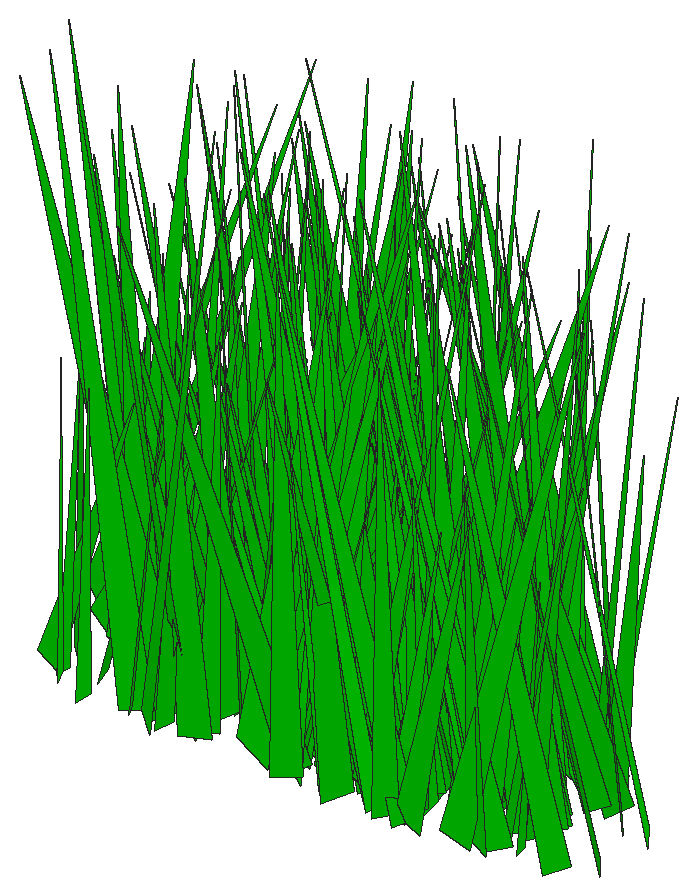
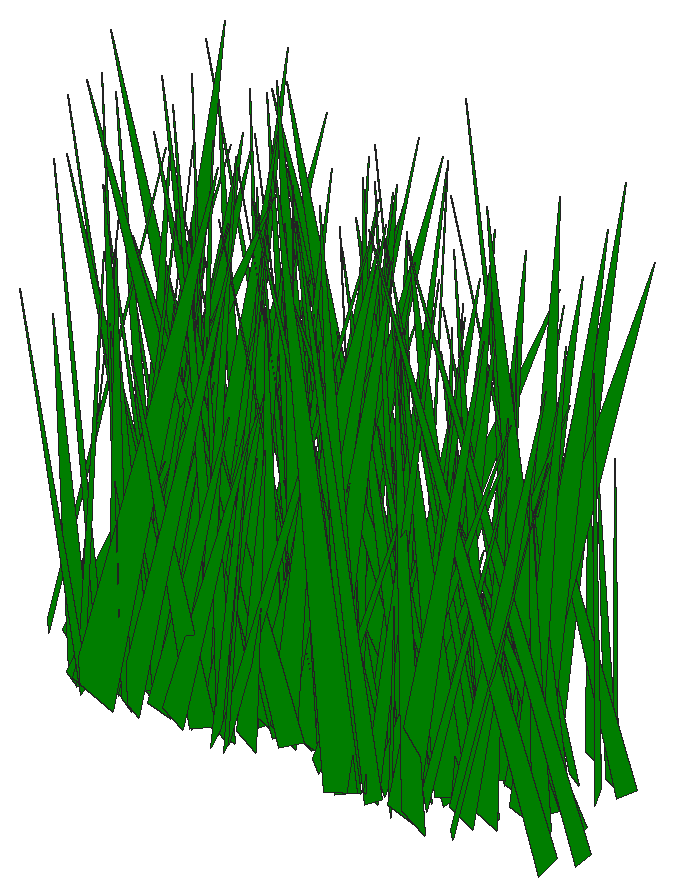
# SketchUp Ruby script. Lengths in inches.
U = 1.inch
M = Sketchup.active_model
def pt(a) = Geom::Point3d.new(a.map { |v| v * U })
def face(e, loops, mat)
  f = e.add_face(loops[0].map { |a| pt(a) })
  loops[1..].each { |l| e.add_face(l.map { |a| pt(a) }).erase! }
  f.material = f.back_material = mat if mat
  f
end
# faces: each face lists its corners as indices into pts; further lists are holes
def faces(e, pts, list, mat = nil) = list.each { |f| face(e, (f[0].is_a?(Array) ? f : [f]).map { |l| l.map { |i| pts[i] } }, mat) }
# xy, xz, yz: faces in a plane at the given z, y or x. An outline is a flat list of corners, or four numbers for a rectangle; further outlines are holes
def ring(l) = l.size == 4 ? [[l[0], l[1]], [l[2], l[1]], [l[2], l[3]], [l[0], l[3]]] : l.each_slice(2).to_a
def flat(e, list, mat, &to3) = list.each { |f| face(e, (f[0].is_a?(Array) ? f : [f]).map { |l| ring(l).map { |u, v| to3.(u, v) } }, mat) }
def xy(e, z, list, mat = nil) = flat(e, list, mat) { |x, y| [x, y, z] }
def xz(e, y, list, mat = nil) = flat(e, list, mat) { |x, z| [x, y, z] }
def yz(e, x, list, mat = nil) = flat(e, list, mat) { |y, z| [x, y, z] }
def lines(e, pts, list) = list.each { |a, b| e.add_line(pt(pts[a]), pt(pts[b])) }
# prism: a flat outline (further loops are holes) pulled along v
def prism(e, loops, v, mat = nil)
  f = face(e, loops, mat); d = Geom::Vector3d.new(v.map { |x| x * U })
  f.pushpull(f.normal.samedirection?(d) ? d.length : -d.length)
end
def box(e, o, s, mat = nil) = prism(e, [[o, [o[0] + s[0], o[1], o[2]], [o[0] + s[0], o[1] + s[1], o[2]], [o[0], o[1] + s[1], o[2]]]], [0, 0, s[2]], mat)
def at(x, y, z, deg = 0) = Geom::Transformation.translation(pt([x, y, z])) * Geom::Transformation.rotation(ORIGIN, Z_AXIS, deg.degrees)
def axes(o, x, y, z) = Geom::Transformation.new([*x, 0, *y, 0, *z, 0, *pt(o).to_a, 1])
def part(name) = M.definitions.add(name)
# library, detail: a bought-in or finely detailed component or shape, given as its bounding box
def library(name, o, s) = part(name).tap { |d| box(d.entities, o, s) }
def detail(e, o, s) = box(e.add_group.entities, o, s)
def put(e, d, t, mat = nil) = e.add_instance(d, t).tap { |i| i.material = mat if mat }
def group(e, t, mat = nil) = e.add_group.tap { |g| g.transformation = t; g.material = mat if mat }.entities
root = M.entities
M.materials.add("[Color G06]").color = [0, 204, 0]
c1 = part("fur_instance\#9")
p = [[0.8125,0,1.79],[0.67,-0.02,1.48],[0,-0.11,0],[0,0.11,0]]
faces(c1.entities,p,[[0,1,2,3]])
put(root,c1,axes([93.32,20.96,4.28],[-4.15856,-0.04522,0.42763],[-0.24087,0.56256,1.60087],[0.35916,-0.14626,6.02509]),"[Color G06]")
put(root,c1,axes([93.11,18.42,4.28],[-1.77363,-0.76487,1.40268],[-5.54361,0.23087,-1.19607],[-0.48553,0.1581,8.53241]),"[Color G06]")
put(root,c1,axes([92.51,19.21,4.28],[-3.03787,0.38662,3.31742],[3.46807,0.41073,1.5953],[0.76567,-0.32643,5.93635]),"[Color G06]")
put(root,c1,axes([91.73,17.29,4.28],[-3.61596,-0.26712,1.95596],[-1.26486,0.5103,2.78243],[1.94484,-0.16477,5.44624]),"[Color G06]")
put(root,c1,axes([91.68,19.55,4.28],[-1.50021,-0.43243,0.52191],[-2.93541,0.21388,1.50933],[1.05913,-0.01973,4.9224]),"[Color G06]")
put(root,c1,axes([91.92,16.38,4.28],[-2.78396,-0.01619,2.16058],[0.38948,0.41195,1.47567],[1.397,-0.14712,3.89424]),"[Color G06]")
put(root,c1,axes([91.82,16.63,4.28],[2.58132,-0.22761,0.58761],[-1.48872,-0.35679,-1.26735],[-0.77617,-0.07262,4.38507]),"[Color G06]")
put(root,c1,axes([92.02,18.39,4.28],[-1.45035,0.39442,0.16935],[2.67143,0.19658,-1.48927],[0.93634,0.05009,4.5113]),"[Color G06]")
put(root,c1,axes([93.66,20.17,4.28],[-2.8666,-0.46823,1.58178],[-3.517,0.37218,-1.58151],[-0.16044,0.20749,6.40624]),"[Color G06]")
put(root,c1,axes([93.95,17.52,4.28],[0.25229,0.76715,0.79622],[5.25095,-0.05648,2.53488],[-1.7254,-0.05972,7.83087]),"[Color G06]")
put(root,c1,axes([91.25,16.77,4.28],[0.7768,-0.41726,0.47828],[-2.7764,-0.08159,1.89573],[1.16095,0.08407,4.21362]),"[Color G06]")
put(root,c1,axes([95.05,16.57,4.28],[-1.07004,0.80814,0.91519],[5.3939,0.10448,3.48938],[-2.20617,-0.13653,8.08736]),"[Color G06]")
put(root,c1,axes([93.05,17.76,4.28],[-2.5649,0.23425,0.39401],[1.54825,0.34923,-1.33748],[0.70304,0.08551,4.38288]),"[Color G06]")
put(root,c1,axes([90.93,19.04,4.28],[2.31582,-0.30652,0.01263],[-1.93543,-0.28352,2.27407],[1.04211,0.1546,4.19539]),"[Color G06]")
put(root,c1,axes([90.05,19.96,4.28],[5.14354,0.39233,0.20234],[2.70873,-0.67815,-2.75667],[0.77264,-0.23431,8.31738]),"[Color G06]")
put(root,c1,axes([94.3,16.24,4.28],[-3.81085,0.59634,1.81684],[4.44015,0.52185,1.127],[0.2262,-0.19697,8.48654]),"[Color G06]")
put(root,c1,axes([93.15,19.87,4.28],[2.44916,-0.44573,0.93395],[-2.98196,-0.35073,-1.7608],[-1.3098,-0.03497,5.75509]),"[Color G06]")
put(root,c1,axes([90.51,20.76,4.28],[5.74425,-0.28536,0.29791],[-2.01718,-0.7662,2.57285],[0.39787,0.2352,8.743]),"[Color G06]")
put(root,c1,axes([92.99,15.9,4.28],[2.57562,-0.26491,0.59469],[-1.71125,-0.35343,-1.53066],[-0.91598,-0.08461,4.53179]),"[Color G06]")
put(root,c1,axes([92.71,18.14,4.28],[-2.36462,0.75183,1.28791],[5.14929,0.35062,-2.39404],[1.81562,-0.01522,8.46708]),"[Color G06]")
put(root,c1,axes([94.37,17.5,4.28],[1.53115,-0.71337,0.51031],[-4.83016,-0.21736,-2.53265],[-1.71957,-0.02464,7.56846]),"[Color G06]")
put(root,c1,axes([94.9,20.03,4.28],[-3.81415,-0.1096,0.77234],[-0.93183,0.48136,-2.43211],[0.1285,0.23741,5.28779]),"[Color G06]")
put(root,c1,axes([94.87,20.97,4.28],[-3.38658,0.46529,1.95903],[3.5822,0.44899,1.58233],[0.13948,-0.23415,6.92708]),"[Color G06]")
put(root,c1,axes([94.38,16.61,4.28],[1.06724,0.74929,1.90632],[5.40058,-0.17948,1.3503],[-1.15494,-0.14687,8.07567]),"[Color G06]")
put(root,c1,axes([93.25,19.56,4.28],[4.75611,-0.26276,1.8293],[-1.75691,-0.68397,-1.08237],[-1.40073,-0.0343,7.56892]),"[Color G06]")
put(root,c1,axes([96.21,20.11,4.28],[-4.19539,-0.22607,0.18995],[-1.56836,0.54953,-2.24485],[-0.42988,0.20147,6.33629]),"[Color G06]")
put(root,c1,axes([96.22,17.75,4.28],[-3.63597,-0.30668,0.22846],[-2.1222,0.47577,-2.07945],[-0.59697,0.17654,6.00089]),"[Color G06]")
put(root,c1,axes([94.35,17.47,4.28],[3.6807,0.05354,2.82113],[0.94083,-0.54532,-1.55298],[-1.68084,-0.18799,5.30843]),"[Color G06]")
put(root,c1,axes([95.64,17.23,4.28],[-1.1041,0.3479,1.4162],[2.57625,0.10162,1.61887],[-0.6966,-0.17561,3.74247]),"[Color G06]")
put(root,c1,axes([94.19,16.15,4.28],[3.40681,0.14764,1.18837],[0.80818,-0.4743,1.59383],[-1.04883,0.11409,5.08817]),"[Color G06]")
put(root,c1,axes([92.7,16.99,4.28],[5.49237,-0.09231,0.12074],[-0.63393,-0.75171,-1.6022],[-0.20697,-0.14711,8.11144]),"[Color G06]")
put(root,c1,axes([96.08,18.93,4.28],[-0.04304,0.39725,0.22765],[2.53975,-0.00434,1.94263],[-1.29945,-0.02164,3.78929]),"[Color G06]")
put(root,c1,axes([93.62,17.48,4.28],[4.23265,-0.12896,1.03424],[-1.06102,-0.57897,1.40614],[-0.45653,0.1499,6.32074]),"[Color G06]")
put(root,c1,axes([95.92,16.22,4.28],[-3.92501,-0.29525,0.5518],[-2.03835,0.54535,1.13373],[0.68158,-0.06933,6.56821]),"[Color G06]")
put(root,c1,axes([94.42,21.09,4.28],[3.80061,-0.41677,0.32666],[-2.77508,-0.50805,-2.33923],[-1.13103,-0.15391,6.83716]),"[Color G06]")
put(root,c1,axes([95.98,20.77,4.28],[-4.91749,0.15917,2.11364],[1.41638,0.6921,1.37353],[1.13877,-0.17348,7.41888]),"[Color G06]")
put(root,c1,axes([96.0625,19.18,4.28],[-4.84141,0.19014,0.95387],[1.11253,0.65377,-2.35708],[1.01431,0.19047,7.13825]),"[Color G06]")
put(root,c1,axes([95.21,19.43,4.28],[2.71413,-0.27368,1.71108],[-1.75241,-0.41044,-1.33229],[-1.44627,-0.01628,4.82537]),"[Color G06]")
put(root,c1,axes([94.52,19.5,4.28],[-0.67718,0.63406,0.19879],[4.44886,0.09622,-1.40461],[0.94912,0.00136,6.72572]),"[Color G06]")
put(root,c1,axes([93.79,19.0625,4.28],[5.0228,0.35797,0.25556],[2.43856,-0.67907,2.20981],[-0.82013,0.1732,8.1358]),"[Color G06]")
put(root,c1,axes([96,18.0625,4.28],[-0.22793,0.54055,2.68699],[4.18813,-0.02154,1.29143],[-0.84767,-0.25179,5.65813]),"[Color G06]")
put(root,c1,axes([94.15,18.125,4.28],[0.89299,-0.56458,0.06541],[-3.97459,-0.12104,1.19653],[0.77259,0.02989,6.07996]),"[Color G06]")
put(root,c1,axes([96.78,18.86,4.28],[2.44031,0.64518,2.4293],[4.02432,-0.40814,3.42196],[-2.80248,-0.02428,7.02925]),"[Color G06]")
put(root,c1,axes([95.33,20.85,4.28],[4.3793,-0.07884,2.83715],[0.27014,-0.61257,-2.88679],[-1.96219,-0.26028,5.93464]),"[Color G06]")
put(root,c1,axes([94.95,19.85,4.28],[3.02987,0.20285,0.89994],[1.31134,-0.42593,1.16666],[-0.87121,0.06434,4.88586]),"[Color G06]")
put(root,c1,axes([95.29,16.05,4.28],[3.25163,0.45455,0.54285],[3.00175,-0.44117,2.27195],[-1.3217,0.11632,6.49542]),"[Color G06]")
put(root,c1,axes([96.18,16.07,4.28],[0.17155,0.64687,1.77041],[4.70831,-0.05278,1.19617],[-0.86854,-0.15834,6.83401]),"[Color G06]")
put(root,c1,axes([94.76,18.55,4.28],[-1.60592,0.64467,2.18363],[4.5724,0.27276,-1.73896],[1.61269,-0.13138,7.10484]),"[Color G06]")
put(root,c1,axes([96.01,17.88,4.28],[-2.75426,0.29226,0.22472],[1.9301,0.36555,-1.77091],[0.83062,0.11968,4.86014]),"[Color G06]")
put(root,c1,axes([97.33,18.375,4.28],[-1.28275,-0.46751,0.11305],[-3.08854,0.1603,-2.13],[-1.30655,0.08007,4.92411]),"[Color G06]")
put(root,c1,axes([94.08,17.98,4.28],[4.007,0.04567,0.15646],[0.34235,-0.51403,-2.34831],[0.032,-0.21954,5.53085]),"[Color G06]")
put(root,c1,axes([96.22,17.62,4.28],[2.95874,-0.67113,0.30492],[-4.43795,-0.39275,-3.11048],[-1.87344,-0.12955,7.8499]),"[Color G06]")
put(root,c1,axes([95.78,18.22,4.28],[2.745,-0.41858,1.48213],[-2.89887,-0.40634,-1.1901],[-1.26111,0.02295,5.96172]),"[Color G06]")
put(root,c1,axes([94.83,15.92,4.28],[5.53723,0.18183,2.45849],[1.71203,-0.76564,-2.1082],[-1.21456,-0.25024,8.23666]),"[Color G06]")
put(root,c1,axes([95.15,19.18,4.28],[0.54778,-0.44335,1.12213],[-3.15104,-0.04369,1.45299],[0.86211,0.12201,4.59774]),"[Color G06]")
put(root,c1,axes([96.51,18.26,4.28],[-5.34507,-0.08397,2.94885],[-0.23534,0.78396,1.61168],[2.04942,-0.12898,7.87593]),"[Color G06]")
put(root,c1,axes([96.71,17.15,4.28],[-4.08381,-0.02123,2.1514],[-0.52777,0.58131,-1.57891],[1.34786,0.1633,5.90019]),"[Color G06]")
put(root,c1,axes([96.29,16.45,4.28],[1.64611,0.4765,0.34657],[3.34245,-0.23133,1.07397],[-0.7474,0.01496,5.56619]),"[Color G06]")
put(root,c1,axes([97.29,18.92,4.28],[-5.45701,0.17626,3.29785],[2.063,0.73278,3.1261],[1.48684,-0.36981,7.7663]),"[Color G06]")
put(root,c1,axes([99.04,16.33,4.28],[-2.73396,-0.61043,0.12845],[-4.05016,0.34722,-3.00448],[-1.66336,0.15787,7.10459]),"[Color G06]")
put(root,c1,axes([98.01,20.36,4.28],[-3.30955,-0.16179,0.09083],[-1.13461,0.44458,-1.37871],[-0.2499,0.12412,5.05692]),"[Color G06]")
put(root,c1,axes([97.95,17.62,4.28],[-2.79481,0.18158,0.23896],[1.2752,0.36367,1.5706],[-0.30815,-0.14186,4.33224]),"[Color G06]")
put(root,c1,axes([97.9,17.74,4.28],[-1.4915,-0.42185,1.28772],[-3.04073,0.15934,-1.87086],[-0.805,0.17973,4.68099]),"[Color G06]")
put(root,c1,axes([95.625,19.05,4.28],[0.95502,0.50004,1.12401],[3.58865,-0.10581,-1.40371],[0.73877,-0.13243,5.36562]),"[Color G06]")
put(root,c1,axes([95.4,19.8,4.28],[4.65554,-0.32798,0.29399],[-2.27103,-0.639,-1.55929],[-0.64281,-0.11783,7.63809]),"[Color G06]")
put(root,c1,axes([94.38,19.51,4.28],[3.04406,0.5202,0.87894],[3.48315,-0.34602,-3.421],[1.45953,-0.25919,6.33101]),"[Color G06]")
put(root,c1,axes([98.27,17.75,4.28],[-1.95236,-0.34271,0.83146],[-2.47148,0.24129,-1.53797],[-0.49138,0.14803,4.43185]),"[Color G06]")
put(root,c1,axes([96.49,18.89,4.28],[5.06297,-0.18053,2.25382],[-1.06562,-0.73234,-1.39143],[-1.67767,-0.07965,7.68551]),"[Color G06]")
put(root,c1,axes([95.81,20.88,4.28],[4.49793,0.34569,2.2561],[2.83354,-0.6071,-1.93267],[-0.62885,-0.26293,7.42864]),"[Color G06]")
put(root,c1,axes([96.76,20.5,4.28],[-3.58448,0.56107,2.40881],[3.82919,0.54656,-1.89621],[2.03075,-0.04026,7.82732]),"[Color G06]")
put(root,c1,axes([96.59,20.99,4.28],[-0.73322,-0.45925,0.49484],[-3.15637,0.11125,1.4137],[0.99678,0.01446,4.84056]),"[Color G06]")
put(root,c1,axes([98.7,19.42,4.28],[0.70035,0.68534,2.16868],[4.82518,-0.15697,2.21758],[-1.72572,-0.16075,7.08055]),"[Color G06]")
put(root,c1,axes([97.58,19.45,4.28],[2.44316,-0.35319,1.3697],[-2.39262,-0.36382,-1.24386],[-1.23718,0.00611,5.11042]),"[Color G06]")
put(root,c1,axes([97.16,19.55,4.28],[4.77282,0.02242,2.53589],[0.59937,-0.68069,-1.82859],[-1.59546,-0.18865,6.89916]),"[Color G06]")
put(root,c1,axes([98.23,17.1,4.28],[1.16702,0.45356,0.2273],[3.04665,-0.16005,1.74612],[-1.14906,0.03629,4.86054]),"[Color G06]")
put(root,c1,axes([96.68,21,4.28],[2.99772,-0.62788,2.49649],[-4.79903,-0.40209,1.25508],[-0.18288,0.25945,7.98655]),"[Color G06]")
put(root,c1,axes([97.1,17.01,4.28],[5.37921,0.10359,2.23831],[0.32036,-0.75452,2.29157],[-1.64076,0.1923,7.7857]),"[Color G06]")
put(root,c1,axes([99.34,19.44,4.28],[1.92923,0.62945,3.47215],[4.4229,-0.37852,2.39345],[-2.49221,-0.1845,6.93542]),"[Color G06]")
put(root,c1,axes([99.33,18.31,4.28],[-2.83966,0.55017,1.09673],[4.00075,0.37828,1.33966],[-0.31444,-0.15547,7.14065]),"[Color G06]")
put(root,c1,axes([97.67,18.75,4.28],[2.84886,0.27506,0.02421],[1.7579,-0.35581,2.31849],[-0.895,0.1767,4.63089]),"[Color G06]")
put(root,c1,axes([100.0625,19.58,4.28],[-0.95755,0.73347,1.72815],[5.15134,0.07698,2.62271],[-1.57074,-0.19468,7.54782]),"[Color G06]")
put(root,c1,axes([100.58,20.7,4.28],[-5.99828,0.07391,0.36249],[0.56482,0.82338,1.59246],[0.14393,-0.15105,8.85779]),"[Color G06]")
put(root,c1,axes([97.31,19.18,4.28],[-0.5576,0.66648,2.24168],[4.79082,0.13243,-1.86114],[1.46345,-0.17959,6.94683]),"[Color G06]")
put(root,c1,axes([96.57,19.59,4.28],[5.62434,-0.0415,1.00254],[-0.52398,-0.73326,3.07983],[-0.51376,0.29358,7.83409]),"[Color G06]")
put(root,c1,axes([99,15.97,4.28],[1.5747,0.65809,0.16988],[4.57999,-0.21703,1.74692],[-1.14401,0.03699,7.22756]),"[Color G06]")
put(root,c1,axes([97.68,16.34,4.28],[-2.28057,0.5941,1.46229],[3.83774,0.34579,-2.76894],[2.09297,0.0133,6.67058]),"[Color G06]")
put(root,c1,axes([98.71,17.22,4.28],[-3.96086,0.53569,1.16906],[3.51831,0.55411,-2.54041],[1.72941,0.0996,7.84569]),"[Color G06]")
put(root,c1,axes([99.58,19.5,4.28],[-3.96788,-0.0309,1.65371],[-0.70523,0.50823,-2.68879],[0.88094,0.26768,5.29607]),"[Color G06]")
put(root,c1,axes([97.43,18.8,4.28],[0.29792,0.38036,0.31023],[2.38196,-0.02175,-2.04601],[1.34523,-0.04572,3.55413]),"[Color G06]")
put(root,c1,axes([99.51,19.73,4.28],[1.37326,0.53249,1.40769],[3.68145,-0.22299,1.66743],[-1.38419,-0.06478,5.83134]),"[Color G06]")
put(root,c1,axes([98.32,18.24,4.28],[2.77066,0.24181,0.28506],[1.64236,-0.37838,1.2138],[-0.5882,0.08249,4.73191]),"[Color G06]")
put(root,c1,axes([100.97,16.83,4.28],[-3.60223,0.59145,2.01635],[4.40953,0.44135,2.72515],[-0.60492,-0.30484,7.85771]),"[Color G06]")
put(root,c1,axes([97.23,17.95,4.28],[2.34243,-0.27021,0.08093],[-1.67827,-0.27676,2.35799],[0.97013,0.17366,3.88378]),"[Color G06]")
put(root,c1,axes([99.64,17.5625,4.28],[4.41423,-0.34648,2.81622],[-2.00437,-0.66411,-2.36823],[-2.38891,-0.08302,7.19082]),"[Color G06]")
put(root,c1,axes([98.62,17.2,4.28],[3.69483,0.22834,0.88536],[1.49492,-0.5153,1.33128],[-0.89302,0.08212,5.89167]),"[Color G06]")
put(root,c1,axes([100.05,16.66,4.28],[-3.218,0.41544,3.08322],[3.54812,0.43942,1.47045],[0.73655,-0.30171,6.38719]),"[Color G06]")
put(root,c1,axes([100.23,19.36,4.28],[-0.12148,0.43098,0.67362],[3.01979,0.00014,1.20602],[-0.79774,-0.06509,4.46275]),"[Color G06]")
put(root,c1,axes([99.01,19.62,4.28],[3.5299,-0.49797,0.80722],[-3.4481,-0.49599,-1.46717],[-1.07454,-0.04426,7.35975]),"[Color G06]")
put(root,c1,axes([98.07,18.33,4.28],[1.5821,-0.42996,1.6831],[-3.16831,-0.15441,2.12109],[0.85865,0.22246,4.72536]),"[Color G06]")
put(root,c1,axes([100.64,17.77,4.28],[-0.07259,-0.68395,2.00154],[-4.92998,-0.0362,-1.82029],[-1.24317,0.18348,7.10176]),"[Color G06]")
put(root,c1,axes([100.55,15.93,4.28],[2.17853,0.72088,0.60462],[4.71913,-0.30098,3.24212],[-2.14909,0.06983,7.73222]),"[Color G06]")
put(root,c1,axes([99.92,16.17,4.28],[-2.85592,0.07121,1.63313],[0.8595,0.39492,1.37937],[0.84618,-0.1608,4.11082]),"[Color G06]")
put(root,c1,axes([99.26,16.03,4.28],[-2.77502,0.15983,1.96077],[0.72823,0.419,-1.62119],[1.58256,0.08745,4.18422]),"[Color G06]")
put(root,c1,axes([97.3,17.07,4.28],[3.17643,0.69279,1.31954],[4.91699,-0.39227,-2.78091],[1.13383,-0.23975,8.36299]),"[Color G06]")
put(root,c1,axes([101.26,17.77,4.28],[-0.56254,0.57765,0.0768],[3.82653,0.06968,2.40389],[-1.58752,-0.03674,5.76707]),"[Color G06]")
put(root,c1,axes([100.08,20.48,4.28],[1.32025,0.42316,0.32196],[2.83011,-0.18285,1.68371],[-1.11601,0.0369,4.65063]),"[Color G06]")
put(root,c1,axes([98.26,16.97,4.28],[-0.03404,0.80754,2.04322],[5.68733,0.06046,-2.53339],[1.7493,-0.18086,8.27632]),"[Color G06]")
put(root,c1,axes([101.41,16.3,4.28],[-1.5489,-0.50915,0.11288],[-3.51755,0.20491,-1.63977],[-0.98187,0.06908,5.69644]),"[Color G06]")
put(root,c1,axes([101.56,16.03,4.28],[-5.24589,0.19209,1.25383],[1.49999,0.72736,1.21736],[0.59287,-0.14054,8.01425]),"[Color G06]")
put(root,c1,axes([100.15,19.39,4.28],[-2.8576,0.50404,0.08045],[3.43534,0.38161,-2.0835],[1.12547,0.11495,6.56386]),"[Color G06]")
put(root,c1,axes([98.53,19.29,4.28],[5.11445,0.14793,0.54653],[0.89589,-0.68159,2.46628],[-0.67569,0.21604,7.40682]),"[Color G06]")
put(root,c1,axes([100.12,18.57,4.28],[-4.65646,0.01506,3.05229],[-0.26024,0.69808,-1.28259],[2.02848,0.12414,6.84213]),"[Color G06]")
put(root,c1,axes([100.24,21.05,4.28],[-2.47169,-0.14679,0.94922],[-0.81067,0.3441,1.39749],[0.92427,-0.09074,3.76414]),"[Color G06]")
put(root,c1,axes([99.22,18.66,4.28],[-1.77969,-0.80274,1.71366],[-5.58807,0.28284,2.25697],[1.79648,0.08457,8.71813]),"[Color G06]")
put(root,c1,axes([99.02,16.43,4.28],[3.50092,0.04389,0.39406],[0.19682,-0.4564,1.93384],[-0.36035,0.17715,4.8846]),"[Color G06]")
put(root,c1,axes([98.43,16.5,4.28],[5.0145,-0.26211,1.89263],[-2.24483,-0.63344,3.20826],[-0.31211,0.3448,7.3326]),"[Color G06]")
put(root,c1,axes([99.37,19.06,4.28],[5.76612,-0.31585,1.45535],[-1.83742,-0.7808,-3.20491],[-1.64397,-0.23516,8.6866]),"[Color G06]")
put(root,c1,axes([98.56,18.89,4.28],[5.37126,0.0041,0.88551],[0.20846,-0.71768,-2.4423],[-0.55538,-0.22968,7.64734]),"[Color G06]")
put(root,c1,axes([100.78,20.75,4.28],[-5.16256,-0.37259,1.15085],[-2.15428,0.67908,3.66936],[1.75822,-0.26196,7.8751]),"[Color G06]")
put(root,c1,axes([99.84,16.58,4.28],[-1.67295,0.60071,0.69439],[4.13229,0.24209,-1.81965],[1.3029,0.00351,6.66284]),"[Color G06]")
put(root,c1,axes([99.87,18,4.28],[2.84654,-0.28088,0.08777],[-1.92169,-0.38263,-1.45016],[-0.60659,-0.10592,5.00598]),"[Color G06]")
put(root,c1,axes([101.24,20.43,4.28],[-0.58315,-0.35266,1.57918],[-2.68465,0.04314,-1.10778],[-0.55229,0.16267,3.71745]),"[Color G06]")
put(root,c1,axes([99.62,18.8,4.28],[4.96815,-0.24595,0.6017],[-1.40256,-0.62725,-3.58534],[-1.14276,-0.29943,7.01634]),"[Color G06]")
put(root,c1,axes([102.55,15.97,4.28],[-3.64773,0.45484,1.14166],[3.32128,0.47041,2.17512],[-0.43819,-0.2209,6.9826]),"[Color G06]")
put(root,c1,axes([101.64,17.57,4.28],[-4.75038,0.16252,2.12012],[1.42109,0.67291,1.18703],[1.16236,-0.1585,7.21334]),"[Color G06]")
put(root,c1,axes([101.52,20.46,4.28],[-5.32779,0.25143,2.02034],[1.556,0.76045,-1.70589],[1.63012,0.09588,8.23151]),"[Color G06]")
put(root,c1,axes([99.12,19.93,4.28],[2.08136,0.54226,0.47024],[3.75825,-0.26533,-2.00968],[1.04713,-0.12555,6.27827]),"[Color G06]")
put(root,c1,axes([99.75,17.87,4.28],[5.2212,-0.00466,1.56552],[0.20783,-0.72287,-1.79532],[-1.02719,-0.16993,7.5943]),"[Color G06]")
put(root,c1,axes([102.16,20.71,4.28],[-0.6846,-0.41077,1.41275],[-2.93397,0.04339,-1.72648],[-0.98111,0.15686,4.1772]),"[Color G06]")
put(root,c1,axes([100.61,20.6,4.28],[2.97573,-0.33653,0.72951],[-2.30335,-0.41821,-1.17438],[-0.86999,-0.04383,5.60448]),"[Color G06]")
put(root,c1,axes([102.16,17.43,4.28],[-0.09027,0.56815,0.2692],[3.9209,0.00518,1.68174],[-1.12222,-0.02761,5.85415]),"[Color G06]")
put(root,c1,axes([102.3,17.88,4.28],[3.40118,0.63637,0.24979],[3.67803,-0.39896,4.89092],[-2.70673,0.25752,6.95988]),"[Color G06]")
put(root,c1,axes([102.15,19.96,4.28],[-0.71687,0.40183,1.23762],[2.92533,0.06771,1.25942],[-0.65725,-0.1369,4.25563]),"[Color G06]")
put(root,c1,axes([102.84,17.59,4.28],[-3.24116,-0.06662,0.1267],[-0.48208,0.43301,-1.3907],[-0.05533,0.13006,4.69486]),"[Color G06]")
put(root,c1,axes([102.68,20.59,4.28],[-1.43867,0.43658,0.08105],[3.05947,0.19421,1.13327],[-0.66699,-0.05086,5.02344]),"[Color G06]")
put(root,c1,axes([103.04,17.89,4.28],[1.73648,0.6151,1.70568],[3.86624,-0.28903,3.18148],[-2.41085,-0.02047,6.33065]),"[Color G06]")
put(root,c1,axes([101.18,18.1875,4.28],[-2.14092,-0.66778,0.01344],[-4.54265,0.28363,2.47587],[1.51581,-0.09319,7.43879]),"[Color G06]")
put(root,c1,axes([100.77,16.66,4.28],[-0.32976,-0.45432,1.37617],[-3.15891,0.0877,1.63527],[1.21819,0.10444,4.613]),"[Color G06]")
put(root,c1,axes([103.4,20.86,4.28],[-3.80778,-0.42771,1.28241],[-3.1843,0.50741,-1.67942],[-0.06533,0.19694,7.11209]),"[Color G06]")
put(root,c1,axes([100.9,20.38,4.28],[5.09944,0.26951,3.14724],[2.5459,-0.70129,-2.31556],[-1.29935,-0.31634,7.8147]),"[Color G06]")
put(root,c1,axes([99.58,19.62,4.28],[2.96934,0.53056,0.15299],[3.61447,-0.38739,-2.37323],[1.19261,-0.14689,6.81168]),"[Color G06]")
put(root,c1,axes([100.26,19.34,4.28],[4.78257,-0.34729,1.68662],[-2.72272,-0.63401,2.2488],[-0.25114,0.25992,7.73892]),"[Color G06]")
put(root,c1,axes([102.86,19.625,4.28],[-2.66011,-0.47533,2.30068],[-3.73133,0.35535,-1.20339],[0.2567,0.23959,6.34922]),"[Color G06]")
put(root,c1,axes([103.4,18.51,4.28],[-3.97889,-0.50809,2.12809],[-3.90269,0.53503,-1.62515],[0.26905,0.247,7.89796]),"[Color G06]")
put(root,c1,axes([101.625,20,4.28],[4.39671,-0.01294,2.35594],[0.3434,-0.62691,-1.82724],[-1.54127,-0.17661,6.31358]),"[Color G06]")
put(root,c1,axes([101.97,15.9375,4.28],[2.80051,-0.48193,0.82493],[-3.29783,-0.39638,-1.59286],[-1.17176,-0.03623,6.4546]),"[Color G06]")
put(root,c1,axes([103.95,17.98,4.28],[-1.72586,-0.56067,0.69081],[-3.84713,0.20551,-2.30848],[-1.25666,0.14084,6.11842]),"[Color G06]")
put(root,c1,axes([103.88,17.13,4.28],[-4.50679,0.1495,0.74662],[1.17113,0.60243,1.93407],[0.16543,-0.19205,6.64806]),"[Color G06]")
put(root,c1,axes([100.63,16.96,4.28],[6.08065,-0.0139,1.62464],[-0.41776,-0.82219,2.68474],[-1.00848,0.2568,8.68365]),"[Color G06]")
put(root,c1,axes([102.66,19.2,4.28],[4.52804,0.38413,2.92861],[2.20706,-0.68189,2.65173],[-2.56061,0.09153,7.4644]),"[Color G06]")
put(root,c1,axes([100.72,17.72,4.28],[4.90633,0.10627,0.38776],[0.57403,-0.61846,3.24715],[-0.56446,0.29479,6.67265]),"[Color G06]")
put(root,c1,axes([101.32,20.6,4.28],[0.17148,0.51869,0.25977],[3.58426,-0.01641,-1.52028],[1.00953,-0.02983,5.35352]),"[Color G06]")
put(root,c1,axes([101.95,19.5,4.28],[5.40063,0.11248,3.36012],[1.32304,-0.78619,-1.72668],[-1.98865,-0.21757,7.97643]),"[Color G06]")
put(root,c1,axes([101.71,18.6,4.28],[-1.18818,0.44175,2.27829],[3.27874,0.22021,-1.08526],[1.26856,-0.15539,4.93892]),"[Color G06]")
put(root,c1,axes([103.51,17.35,4.28],[-4.26816,0.54302,2.63827],[4.21731,0.59191,1.245],[0.70334,-0.2539,8.54494]),"[Color G06]")
put(root,c1,axes([103.53,17.98,4.28],[0.67869,0.51892,1.88919],[3.62977,-0.15134,1.86271],[-1.50686,-0.13084,5.33782]),"[Color G06]")
put(root,c1,axes([100.97,17.47,4.28],[3.93324,0.13226,0.61901],[1.02994,-0.52256,-1.79203],[-0.10199,-0.17632,5.7754]),"[Color G06]")
put(root,c1,axes([103.64,19.94,4.28],[-2.5224,-0.29047,1.3378],[-2.26533,0.31526,-1.67751],[-0.09268,0.19977,4.59246]),"[Color G06]")
put(root,c1,axes([101.83,18.125,4.28],[4.72892,-0.42584,1.04828],[-2.82786,-0.6563,-2.1308],[-1.3494,-0.11697,8.13902]),"[Color G06]")
put(root,c1,axes([102.61,16.8,4.28],[2.76427,-0.33055,0.49279],[-1.99729,-0.35732,-2.50699],[-1.31855,-0.15172,4.83063]),"[Color G06]")
put(root,c1,axes([104.56,16.75,4.28],[-4.74363,0.42826,1.10259],[3.15757,0.63838,1.86077],[-0.07832,-0.20151,8.23836]),"[Color G06]")
put(root,c1,axes([102.46,16.73,4.28],[4.62901,0.29648,2.64156],[1.98401,-0.69094,1.14233],[-1.92561,0.00081,7.52707]),"[Color G06]")
put(root,c1,axes([103.47,19.57,4.28],[-3.32548,0.19874,1.63157],[1.69487,0.4532,1.37506],[0.59186,-0.18117,5.22963]),"[Color G06]")
put(root,c1,axes([104.43,20.97,4.28],[-0.97501,-0.81036,0.49355],[-5.62718,0.11929,-2.33154],[-1.48822,0.07984,8.49254]),"[Color G06]")
put(root,c1,axes([102.14,16.1,4.28],[-1.13118,0.36186,0.94589],[2.40428,0.17969,-1.47432],[1.16364,-0.01951,3.9657]),"[Color G06]")
put(root,c1,axes([103.66,20.25,4.28],[-4.35678,-0.35246,0.0303],[-2.25996,0.5457,3.32487],[1.13209,-0.26706,6.75395]),"[Color G06]")
put(root,c1,axes([103.71,18.89,4.28],[-3.71782,0.29153,0.79383],[1.94318,0.51672,-1.47068],[0.93651,0.0852,6.20289]),"[Color G06]")
put(root,c1,axes([103.03,19.6,4.28],[2.98027,-0.22499,0.92878],[-1.16923,-0.38947,-2.45741],[-1.27371,-0.16891,4.42903]),"[Color G06]")
put(root,c1,axes([106.125,19.49,4.28],[-3.63803,-0.63975,0.07813],[-4.26226,0.46781,-3.29639],[-1.69815,0.19639,8.1064]),"[Color G06]")
put(root,c1,axes([105.04,16.37,4.28],[-2.42151,0.47136,0.2756],[3.29429,0.32083,1.62204],[-0.77946,-0.1084,5.99914]),"[Color G06]")
put(root,c1,axes([104.53,19.85,4.28],[-5.15265,0.19445,0.89085],[1.08908,0.67933,-2.96302],[1.05532,0.24835,7.4074]),"[Color G06]")
put(root,c1,axes([100.87,19.34,4.28],[4.17115,-0.59368,0.60969],[-4.16448,-0.54567,2.60392],[0.9744,0.20928,8.51894]),"[Color G06]")
put(root,c1,axes([105.4,17.89,4.28],[-1.65997,0.71263,1.29959],[5.02886,0.19046,2.35063],[-1.25844,-0.17891,7.6791]),"[Color G06]")
put(root,c1,axes([105.1,17.44,4.28],[-0.40971,0.80757,0.10582],[5.59983,0.05271,2.22239],[-1.47854,-0.02415,8.38774]),"[Color G06]")
put(root,c1,axes([102.61,15.97,4.28],[0.23498,-0.49121,0.0491],[-3.34666,-0.02969,1.6505],[1.09985,0.01459,5.01171]),"[Color G06]")
put(root,c1,axes([104.08,19.03,4.28],[2.41144,-0.31719,0.09477],[-1.73133,-0.26411,-3.13804],[-1.47666,-0.20833,3.83399]),"[Color G06]")
put(root,c1,axes([104.79,18.95,4.28],[-5.24028,-0.01813,1.90607],[-0.4588,0.72535,-2.0251],[1.19702,0.19866,7.56813]),"[Color G06]")
put(root,c1,axes([103.99,20.52,4.28],[-3.79577,0.40302,1.11542],[2.56147,0.52622,-2.37077],[1.53264,0.11867,6.72472]),"[Color G06]")
put(root,c1,axes([105.64,19.28,4.28],[-1.29924,-0.55662,0.51129],[-3.75685,0.15185,-2.33393],[-1.39156,0.10973,5.82362]),"[Color G06]")
put(root,c1,axes([102.81,17.74,4.28],[0.72481,-0.35265,0.94649],[-2.4646,-0.06281,1.52762],[0.84985,0.11861,3.62293]),"[Color G06]")
put(root,c1,axes([105.32,20.67,4.28],[-2.53683,0.15999,0.05308],[1.07356,0.32643,1.58234],[-0.40639,-0.13641,3.84864]),"[Color G06]")
put(root,c1,axes([103.69,20.25,4.28],[-2.67406,0.62436,0.84635],[4.25527,0.37938,-2.11882],[1.50371,0.03672,7.50099]),"[Color G06]")
put(root,c1,axes([105.43,18.37,4.28],[-4.44376,0.12428,0.95178],[1.02747,0.60153,1.69266],[0.37969,-0.17327,6.55889]),"[Color G06]")
put(root,c1,axes([104.2,19.49,4.28],[-2.43472,0.10275,1.91123],[1.20309,0.33742,1.33964],[0.85486,-0.18224,3.55802]),"[Color G06]")
put(root,c1,axes([103.48,20.85,4.28],[5.58317,-0.15363,2.63916],[-0.74595,-0.8058,-1.86361],[-1.94308,-0.1321,8.2987]),"[Color G06]")
put(root,c1,axes([104.85,17.96,4.28],[-3.93402,-0.21641,1.9524],[-1.83183,0.54974,-1.2452],[0.87139,0.17865,6.19678]),"[Color G06]")
put(root,c1,axes([103.33,17.07,4.28],[0.35071,0.40863,0.90186],[2.91266,-0.02727,-1.11084],[0.68385,-0.09343,4.26876]),"[Color G06]")
put(root,c1,axes([104.6,19.03,4.28],[3.7754,-0.36588,2.87216],[-2.43534,-0.59017,-1.48584],[-2.15564,0.02593,6.70894]),"[Color G06]")
put(root,c1,axes([105.32,17.77,4.28],[1.70253,-0.77828,3.05668],[-5.59767,-0.30973,-2.09486],[-1.99987,0.20437,8.46576]),"[Color G06]")
put(root,c1,axes([103.15,18.89,4.28],[1.09982,0.41876,0.39283],[2.92544,-0.13885,-1.29215],[0.72755,-0.07473,4.60187]),"[Color G06]")
put(root,c1,axes([102.93,17.5,4.28],[5.03066,-0.39663,0.0567],[-2.733,-0.67691,-2.29887],[-0.78889,-0.1842,8.3257]),"[Color G06]")
put(root,c1,axes([102.67,19.7,4.28],[4.80723,-0.2179,1.17817],[-1.72745,-0.64234,2.09748],[-0.28114,0.22101,7.25779]),"[Color G06]")
put(root,c1,axes([104.53,16.14,4.28],[-2.05826,-0.4049,0.46374],[-2.77229,0.28757,1.35807],[0.91761,-0.03942,5.14317]),"[Color G06]")
put(root,c1,axes([103.35,19.23,4.28],[4.484,0.11996,1.56981],[1.18215,-0.59352,-2.33255],[-0.66766,-0.24525,6.41284]),"[Color G06]")
put(root,c1,axes([104.96,20.8,4.28],[-3.74858,-0.21983,1.77612],[-1.38334,0.5462,1.24426],[1.40848,-0.04861,5.94907]),"[Color G06]")
put(root,c1,axes([103.41,19.75,4.28],[5.01997,0.25848,1.56285],[2.01145,-0.69829,-1.16493],[-0.69538,-0.15386,7.91257]),"[Color G06]")
put(root,c1,axes([104.26,16.85,4.28],[0.18528,-0.41473,1.85358],[-3.14717,0.01391,1.06034],[0.69208,0.17431,4.32564]),"[Color G06]")
put(root,c1,axes([106.73,16.38,4.28],[-2.71734,0.47339,1.75602],[3.55044,0.32262,2.28169],[-0.54711,-0.25757,6.08528]),"[Color G06]")
put(root,c1,axes([107.4,17.15,4.28],[-5.52358,-0.07679,0.28304],[-0.58233,0.72861,-2.67709],[0.00056,0.25117,7.85252]),"[Color G06]")
put(root,c1,axes([105.51,16.57,4.28],[2.23612,0.21835,0.49275],[1.3551,-0.30041,1.55559],[-0.85102,0.09537,3.77176]),"[Color G06]")
put(root,c1,axes([104.74,20.9,4.28],[3.67688,-0.05252,1.122],[-0.54447,-0.50698,1.2596],[-0.63951,0.12968,5.3786]),"[Color G06]")
put(root,c1,axes([104.8125,16.93,4.28],[3.10509,0.13931,1.15769],[1.2118,-0.40958,-1.59841],[-0.35995,-0.17717,4.60558]),"[Color G06]")
put(root,c1,axes([107.4,18.97,4.28],[-5.31166,-0.06958,0.66772],[-0.35113,0.71337,2.30001],[0.57033,-0.20882,7.6347]),"[Color G06]")
put(root,c1,axes([105.36,17.26,4.28],[4.22485,0.41932,1.32],[2.81793,-0.59872,1.70184],[-1.37178,0.06155,7.5613]),"[Color G06]")
put(root,c1,axes([105.25,19.625,4.28],[4.29877,0.26548,1.54808],[1.76508,-0.61501,1.16739],[-1.2578,0.0443,6.92908]),"[Color G06]")
put(root,c1,axes([105.34,20.29,4.28],[-0.32307,-0.47434,0.6159],[-3.33918,0.05653,1.08895],[0.76866,0.04622,4.98942]),"[Color G06]")
put(root,c1,axes([103.95,16.05,4.28],[4.1655,-0.4976,0.73173],[-3.58769,-0.56395,1.56595],[0.3194,0.155,8.04678]),"[Color G06]")
put(root,c1,axes([106.43,19.18,4.28],[-4.26338,-0.17487,1.47813],[-0.73104,0.5632,2.94417],[1.41998,-0.23509,5.95368]),"[Color G06]")
